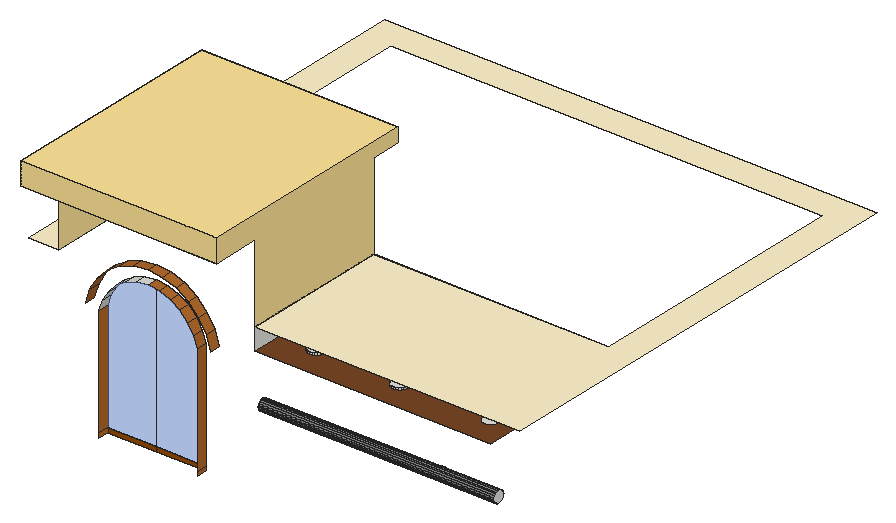
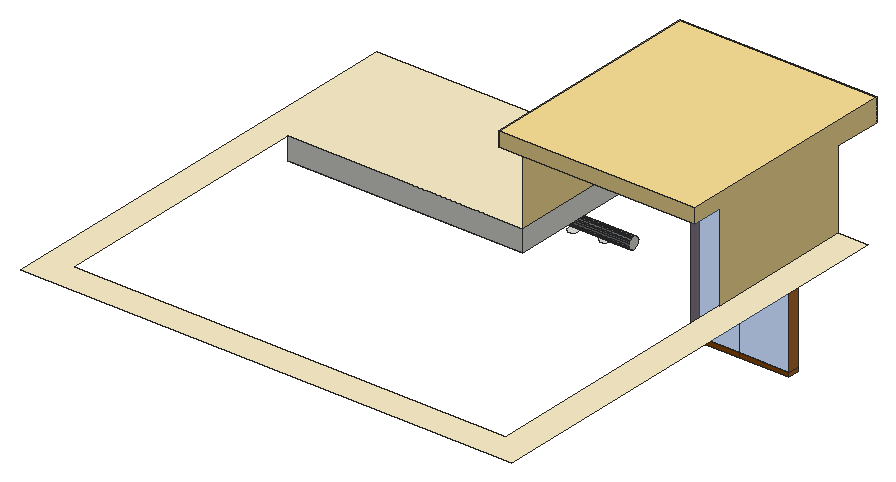
# SketchUp Ruby script. Lengths in inches.
U = 1.inch
M = Sketchup.active_model
def pt(a) = Geom::Point3d.new(a.map { |v| v * U })
def face(e, loops, mat)
  f = e.add_face(loops[0].map { |a| pt(a) })
  loops[1..].each { |l| e.add_face(l.map { |a| pt(a) }).erase! }
  f.material = f.back_material = mat if mat
  f
end
# faces: each face lists its corners as indices into pts; further lists are holes
def faces(e, pts, list, mat = nil) = list.each { |f| face(e, (f[0].is_a?(Array) ? f : [f]).map { |l| l.map { |i| pts[i] } }, mat) }
# xy, xz, yz: faces in a plane at the given z, y or x. An outline is a flat list of corners, or four numbers for a rectangle; further outlines are holes
def ring(l) = l.size == 4 ? [[l[0], l[1]], [l[2], l[1]], [l[2], l[3]], [l[0], l[3]]] : l.each_slice(2).to_a
def flat(e, list, mat, &to3) = list.each { |f| face(e, (f[0].is_a?(Array) ? f : [f]).map { |l| ring(l).map { |u, v| to3.(u, v) } }, mat) }
def xy(e, z, list, mat = nil) = flat(e, list, mat) { |x, y| [x, y, z] }
def xz(e, y, list, mat = nil) = flat(e, list, mat) { |x, z| [x, y, z] }
def yz(e, x, list, mat = nil) = flat(e, list, mat) { |y, z| [x, y, z] }
def lines(e, pts, list) = list.each { |a, b| e.add_line(pt(pts[a]), pt(pts[b])) }
# prism: a flat outline (further loops are holes) pulled along v
def prism(e, loops, v, mat = nil)
  f = face(e, loops, mat); d = Geom::Vector3d.new(v.map { |x| x * U })
  f.pushpull(f.normal.samedirection?(d) ? d.length : -d.length)
end
def box(e, o, s, mat = nil) = prism(e, [[o, [o[0] + s[0], o[1], o[2]], [o[0] + s[0], o[1] + s[1], o[2]], [o[0], o[1] + s[1], o[2]]]], [0, 0, s[2]], mat)
def at(x, y, z, deg = 0) = Geom::Transformation.translation(pt([x, y, z])) * Geom::Transformation.rotation(ORIGIN, Z_AXIS, deg.degrees)
def axes(o, x, y, z) = Geom::Transformation.new([*x, 0, *y, 0, *z, 0, *pt(o).to_a, 1])
def part(name) = M.definitions.add(name)
# library, detail: a bought-in or finely detailed component or shape, given as its bounding box
def library(name, o, s) = part(name).tap { |d| box(d.entities, o, s) }
def detail(e, o, s) = box(e.add_group.entities, o, s)
def put(e, d, t, mat = nil) = e.add_instance(d, t).tap { |i| i.material = mat if mat }
def group(e, t, mat = nil) = e.add_group.tap { |g| g.transformation = t; g.material = mat if mat }.entities
root = M.entities
M.materials.add("[Blacktop Old 01]").color = [132, 136, 139]
M.materials.add("[Color C07]").color = [153, 76, 0]
M.materials.add("[Color D01]").color = [255, 242, 204]
M.materials.add("[Color D02]").color = [255, 229, 153]
M.materials.add("[Translucent Glass Blue]").color = [100, 149, 237]
M.materials["[Translucent Glass Blue]"].alpha = 0.5
M.materials.add("[Wood Bamboo]").color = [177, 105, 43]
M.materials.add("[Wood Veneer 01]").color = [120, 70, 37]
xy(root,265.4375,[[117.93,77.67,118.3,77.72,118.65,77.86,118.94,78.09,119.17,78.39,119.32,78.73,119.36,79.11,119.32,79.48,119.17,79.83,118.94,80.12,118.65,80.35,118.3,80.5,117.93,80.54,117.56,80.5,117.21,80.35,116.91,80.12,116.68,79.83,116.54,79.48,116.49,79.11,116.54,78.73,116.68,78.39,116.91,78.09,117.21,77.86,117.56,77.72]])
xy(root,265.9375,[[129.74,77.67,130.11,77.72,130.46,77.86,130.76,78.09,130.98,78.39,131.13,78.73,131.18,79.11,131.13,79.48,130.98,79.83,130.76,80.12,130.46,80.35,130.11,80.5,129.74,80.54,129.37,80.5,129.02,80.35,128.72,80.12,128.49,79.83,128.35,79.48,128.3,79.11,128.35,78.73,128.49,78.39,128.72,78.09,129.02,77.86,129.37,77.72]])
xy(root,266.15,[[108.24,77.67,108.61,77.72,108.96,77.86,109.26,78.09,109.48,78.39,109.63,78.73,109.68,79.09,106.8,79.09,106.85,78.73,106.99,78.39,107.22,78.09,107.52,77.86,107.87,77.72],[106.8,79.09,109.68,79.09,109.68,79.11,109.63,79.48,109.48,79.83,109.26,80.12,108.96,80.35,108.61,80.5,108.24,80.54,107.87,80.5,107.52,80.35,107.22,80.12,106.99,79.83,106.85,79.48,106.8,79.11]])
xy(root,266.3125,[[141.86,77.67,142.24,77.72,142.58,77.86,142.88,78.09,143.11,78.39,143.25,78.73,143.3,79.11,143.25,79.48,143.11,79.83,142.88,80.12,142.58,80.35,142.24,80.5,141.86,80.54,141.49,80.5,141.15,80.35,140.85,80.12,140.62,79.83,140.48,79.48,140.43,79.11,140.48,78.73,140.62,78.39,140.85,78.09,141.15,77.86,141.49,77.72]])
xy(root,266.75,[[164.61,77.67,164.99,77.72,165.33,77.86,165.63,78.09,165.86,78.39,166,78.73,166.05,79.11,166,79.48,165.86,79.83,165.63,80.12,165.33,80.35,164.99,80.5,164.61,80.54,164.24,80.5,163.9,80.35,163.6,80.12,163.37,79.83,163.23,79.48,163.18,79.11,163.23,78.73,163.37,78.39,163.6,78.09,163.9,77.86,164.24,77.72]])
xy(root,267.84,[[153.24,77.67,153.61,77.72,153.96,77.86,154.26,78.09,154.48,78.39,154.63,78.73,154.68,79.11,154.63,79.48,154.6,79.54,151.88,79.54,151.85,79.48,151.8,79.11,151.85,78.73,151.99,78.39,152.22,78.09,152.52,77.86,152.87,77.72],[151.88,79.54,154.6,79.54,154.48,79.83,154.26,80.12,153.96,80.35,153.61,80.5,153.24,80.54,152.87,80.5,152.52,80.35,152.22,80.12,151.99,79.83]])
xy(root,283.17,[[165.02,81.32,164.35,81.41,163.73,81.66,163.2,82.07,162.8,82.6,162.54,83.22,162.45,83.88,162.54,84.55,162.8,85.16,163.2,85.69,163.73,86.1,164.35,86.36,165.02,86.44,165.68,86.36,166.3,86.1,166.83,85.69,167.24,85.16,167.49,84.55,167.58,83.88,167.49,83.22,167.24,82.6,166.83,82.07,166.3,81.66,165.68,81.41],[165.02,104.69,164.35,104.78,163.73,105.04,163.2,105.45,162.8,105.98,162.54,106.59,162.45,107.26,162.54,107.92,162.8,108.54,163.2,109.07,163.73,109.48,164.35,109.73,165.02,109.82,165.68,109.73,166.3,109.48,166.83,109.07,167.24,108.54,167.49,107.92,167.58,107.26,167.49,106.59,167.24,105.98,166.83,105.45,166.3,105.04,165.68,104.78]])
xy(root,283.17,[[[100.51,74.84,172.07,119.85],[165.02,104.69,165.68,104.78,166.3,105.04,166.83,105.45,167.24,105.98,167.49,106.59,167.58,107.26,167.49,107.92,167.24,108.54,166.83,109.07,166.3,109.48,165.68,109.73,165.02,109.82,164.35,109.73,163.73,109.48,163.2,109.07,162.8,108.54,162.54,107.92,162.45,107.26,162.54,106.59,162.8,105.98,163.2,105.45,163.73,105.04,164.35,104.78],[111.45,82.07,112.12,82.16,112.73,82.41,113.27,82.82,113.67,83.35,113.93,83.97,114.02,84.63,113.93,85.3,113.67,85.91,113.27,86.44,112.73,86.85,112.12,87.11,111.45,87.19,110.79,87.11,110.17,86.85,109.64,86.44,109.23,85.91,108.98,85.3,108.89,84.63,108.98,83.97,109.23,83.35,109.64,82.82,110.17,82.41,110.79,82.16],[111.45,104.69,112.12,104.78,112.73,105.04,113.27,105.45,113.67,105.98,113.93,106.59,114.02,107.26,113.93,107.92,113.67,108.54,113.27,109.07,112.73,109.48,112.12,109.73,111.45,109.82,110.79,109.73,110.17,109.48,109.64,109.07,109.23,108.54,108.98,107.92,108.89,107.26,108.98,106.59,109.23,105.98,109.64,105.45,110.17,105.04,110.79,104.78],[165.02,81.32,165.68,81.41,166.3,81.66,166.83,82.07,167.24,82.6,167.49,83.22,167.58,83.88,167.49,84.55,167.24,85.16,166.83,85.69,166.3,86.1,165.68,86.36,165.02,86.44,164.35,86.36,163.73,86.1,163.2,85.69,162.8,85.16,162.54,84.55,162.45,83.88,162.54,83.22,162.8,82.6,163.2,82.07,163.73,81.66,164.35,81.41],[137.45,81.32,138.12,81.41,138.73,81.66,139.27,82.07,139.67,82.6,139.93,83.22,140.02,83.88,139.93,84.55,139.67,85.16,139.27,85.69,138.73,86.1,138.12,86.36,137.45,86.44,136.79,86.36,136.17,86.1,135.64,85.69,135.23,85.16,134.98,84.55,134.89,83.88,134.98,83.22,135.23,82.6,135.64,82.07,136.17,81.66,136.79,81.41],[137.45,105.26,138.12,105.34,138.73,105.6,139.27,106.01,139.67,106.54,139.93,107.16,140.02,107.82,139.93,108.48,139.67,109.1,139.27,109.63,138.73,110.04,138.12,110.3,137.45,110.38,136.79,110.3,136.17,110.04,135.64,109.63,135.23,109.1,134.98,108.48,134.89,107.82,134.98,107.16,135.23,106.54,135.64,106.01,136.17,105.6,136.79,105.34]]],"[Wood Veneer 01]")
xy(root,283.61,[[137.45,81.32,136.79,81.41,136.17,81.66,135.64,82.07,135.23,82.6,134.98,83.22,134.89,83.88,134.98,84.55,135.23,85.16,135.64,85.69,136.17,86.1,136.79,86.36,137.45,86.44,138.12,86.36,138.73,86.1,139.27,85.69,139.67,85.16,139.93,84.55,140.02,83.88,139.93,83.22,139.67,82.6,139.27,82.07,138.73,81.66,138.12,81.41],[111.45,82.07,110.79,82.16,110.17,82.41,109.64,82.82,109.23,83.35,108.98,83.97,108.89,84.63,108.98,85.3,109.23,85.91,109.64,86.44,110.17,86.85,110.79,87.11,111.45,87.19,112.12,87.11,112.73,86.85,113.27,86.44,113.67,85.91,113.93,85.3,114.02,84.63,113.93,83.97,113.67,83.35,113.27,82.82,112.73,82.41,112.12,82.16],[111.45,104.69,110.79,104.78,110.17,105.04,109.64,105.45,109.23,105.98,108.98,106.59,108.89,107.26,108.98,107.92,109.23,108.54,109.64,109.07,110.17,109.48,110.79,109.73,111.45,109.82,112.12,109.73,112.73,109.48,113.27,109.07,113.67,108.54,113.93,107.92,114.02,107.26,113.93,106.59,113.67,105.98,113.27,105.45,112.73,105.04,112.12,104.78]])
xy(root,283.86,[[137.45,105.26,136.79,105.34,136.17,105.6,135.64,106.01,135.23,106.54,134.98,107.16,134.89,107.82,134.98,108.48,135.23,109.1,135.64,109.63,136.17,110.04,136.79,110.3,137.45,110.38,138.12,110.3,138.73,110.04,139.27,109.63,139.67,109.1,139.93,108.48,140.02,107.82,139.93,107.16,139.67,106.54,139.27,106.01,138.73,105.6,138.12,105.34]])
xy(root,289.8125,[[31.82,74.84,40.82,74.84,40.82,201.03,172.07,201.03,172.07,119.85,100.51,119.85,100.51,74.84,181.07,74.84,181.07,210.03,31.82,210.03]],"[Color D01]")
xy(root,313.4,[[40.82,60.4,100.51,74.84]])
xy(root,315.96,[[40.82,119.85,100.51,129.15]])
xy(root,320.375,[[40.82,60.4,100.51,129.15]],"[Color D02]")
xz(root,60.4,[[40.82,313.4,100.51,320.375]],"[Color D02]")
xz(root,74.84,[[55.76,245.31,70.65,246.56],[70.65,245.31,85.54,246.56]],"[Color C07]")
xz(root,74.84,[[55.76,246.56,70.65,246.56,70.65,292.04,67.19,291.64,63.91,290.47,60.98,288.58,58.5625,286.07,56.77,283.08,55.76,279.92],[70.65,246.56,85.54,246.56,85.54,279.92,84.53,283.08,82.74,286.07,80.32,288.58,77.39,290.47,74.11,291.64,70.65,292.04]],"[Translucent Glass Blue]")
xz(root,119.85,[[100.51,283.17,172.07,289.8125]])
xz(root,129.15,[[40.82,315.96,100.51,320.375]],"[Color D02]")
yz(root,40.82,[[74.84,289.8125,119.85,289.8125,119.85,315.96,129.15,315.96,129.15,320.375,60.4,320.375,60.4,313.4,74.84,313.4]],"[Color D02]")
yz(root,55.76,[[71.71,245.31,74.84,246.56],[71.71,246.56,74.84,279.92]],"[Wood Bamboo]")
yz(root,85.54,[[71.71,245.31,74.84,246.56],[71.71,246.56,74.84,279.92]],"[Wood Bamboo]")
yz(root,100.51,[[77.85,265.64,77.4,265.7,76.98,265.87,76.62,266.15,76.34,266.51,76.16,266.93,76.1,267.39,76.16,267.84,76.34,268.26,76.62,268.625,76.98,268.9,77.4,269.08,77.85,269.14,78.31,269.08,78.73,268.9,79.09,268.625,79.37,268.26,79.54,267.84,79.6,267.39,79.54,266.93,79.37,266.51,79.09,266.15,78.73,265.87,78.31,265.7],[74.84,283.17,119.85,289.8125]])
yz(root,100.51,[[74.84,289.8125,119.85,289.8125,119.85,315.96,129.15,315.96,129.15,320.375,60.4,320.375,60.4,313.4,74.84,313.4]],"[Color D02]")
yz(root,172.14,[[77.85,265.64,78.31,265.7,78.73,265.87,79.09,266.15,79.37,266.51,79.54,266.93,79.6,267.39,79.54,267.84,79.37,268.26,79.09,268.625,78.73,268.9,78.31,269.08,77.85,269.14,77.4,269.08,76.98,268.9,76.62,268.625,76.34,268.26,76.16,267.84,76.1,267.39,76.16,266.93,76.34,266.51,76.62,266.15,76.98,265.87,77.4,265.7]])
p = [[100.51,77.4,265.7],[100.51,77.85,265.64],[172.14,77.85,265.64],[172.14,77.4,265.7],[100.51,78.31,265.7],[172.14,78.31,265.7],
  [100.51,76.98,265.87],[172.14,76.98,265.87],[100.51,78.73,265.87],[172.14,78.73,265.87],[100.51,76.62,266.15],[172.14,76.62,266.15],
  [100.51,79.09,266.15],[106.8,79.09,266.15],[109.68,79.09,266.15],[172.14,79.09,266.15],[100.51,76.34,266.51],[172.14,76.34,266.51],
  [100.51,79.37,266.51],[172.14,79.37,266.51],[100.51,76.16,266.93],[172.14,76.16,266.93],[100.51,79.54,266.93],[172.14,79.54,266.93],
  [100.51,76.1,267.39],[172.14,76.1,267.39],[100.51,79.6,267.39],[172.14,79.6,267.39],[100.51,76.16,267.84],[172.14,76.16,267.84],
  [100.51,79.54,267.84],[151.88,79.54,267.84],[154.6,79.54,267.84],[172.14,79.54,267.84],[100.51,76.34,268.26],[172.14,76.34,268.26],
  [100.51,79.37,268.26],[172.14,79.37,268.26],[100.51,76.62,268.625],[172.14,76.62,268.625],[100.51,79.09,268.625],[172.14,79.09,268.625],
  [100.51,76.98,268.9],[172.14,76.98,268.9],[100.51,78.73,268.9],[172.14,78.73,268.9],[100.51,77.4,269.08],[172.14,77.4,269.08],
  [100.51,78.31,269.08],[172.14,78.31,269.08],[100.51,77.85,269.14],[172.14,77.85,269.14],[55.76,74.84,279.92],[56.77,74.84,283.08],
  [56.77,71.71,283.08],[55.76,71.71,279.92],[84.53,74.84,283.08],[85.54,74.84,279.92],[85.54,71.71,279.92],[84.53,71.71,283.08],
  [53,74.84,284.79],[51.65,74.84,280.57],[51.65,71.71,280.57],[53,71.71,284.79],[89.65,74.84,280.57],[88.3,74.84,284.79],
  [88.3,71.71,284.79],[89.65,71.71,280.57],[58.5625,74.84,286.07],[58.5625,71.71,286.07],[82.74,74.84,286.07],[82.74,71.71,286.07],
  [137.45,81.32,283.17],[136.79,81.41,283.17],[136.79,81.41,283.61],[137.45,81.32,283.61],[138.12,81.41,283.17],[138.12,81.41,283.61],
  [136.17,81.66,283.17],[136.17,81.66,283.61],[138.73,81.66,283.17],[138.73,81.66,283.61],[135.64,82.07,283.17],[135.64,82.07,283.61],
  [139.27,82.07,283.17],[139.27,82.07,283.61],[111.45,82.07,283.17],[110.79,82.16,283.17],[110.79,82.16,283.61],[111.45,82.07,283.61],
  [112.12,82.16,283.17],[112.12,82.16,283.61],[135.23,82.6,283.17],[135.23,82.6,283.61],[139.67,82.6,283.17],[139.67,82.6,283.61],
  [110.17,82.41,283.17],[110.17,82.41,283.61],[112.73,82.41,283.17],[112.73,82.41,283.61],[109.64,82.82,283.17],[109.64,82.82,283.61],
  [113.27,82.82,283.17],[113.27,82.82,283.61],[134.98,83.22,283.17],[134.98,83.22,283.61],[139.93,83.22,283.17],[139.93,83.22,283.61],
  [109.23,83.35,283.17],[109.23,83.35,283.61],[113.67,83.35,283.17],[113.67,83.35,283.61],[134.89,83.88,283.17],[134.89,83.88,283.61],
  [140.02,83.88,283.17],[140.02,83.88,283.61],[108.98,83.97,283.17],[108.98,83.97,283.61],[113.93,83.97,283.17],[113.93,83.97,283.61],
  [134.98,84.55,283.17],[134.98,84.55,283.61],[139.93,84.55,283.17],[139.93,84.55,283.61],[108.89,84.63,283.17],[108.89,84.63,283.61],
  [114.02,84.63,283.17],[114.02,84.63,283.61],[135.23,85.16,283.17],[135.23,85.16,283.61],[139.67,85.16,283.17],[139.67,85.16,283.61],
  [108.98,85.3,283.17],[108.98,85.3,283.61],[113.93,85.3,283.17],[113.93,85.3,283.61],[135.64,85.69,283.17],[135.64,85.69,283.61],
  [139.27,85.69,283.17],[139.27,85.69,283.61],[109.23,85.91,283.17],[109.23,85.91,283.61],[113.67,85.91,283.17],[113.67,85.91,283.61],
  [136.17,86.1,283.17],[136.17,86.1,283.61],[138.73,86.1,283.17],[138.73,86.1,283.61],[109.64,86.44,283.17],[109.64,86.44,283.61],
  [113.27,86.44,283.17],[113.27,86.44,283.61],[136.79,86.36,283.17],[136.79,86.36,283.61],[138.12,86.36,283.17],[138.12,86.36,283.61],
  [110.17,86.85,283.17],[110.17,86.85,283.61],[112.73,86.85,283.17],[112.73,86.85,283.61],[137.45,86.44,283.17],[137.45,86.44,283.61],
  [110.79,87.11,283.17],[110.79,87.11,283.61],[112.12,87.11,283.17],[112.12,87.11,283.61],[111.45,87.19,283.17],[111.45,87.19,283.61],
  [111.45,104.69,283.17],[110.79,104.78,283.17],[110.79,104.78,283.61],[111.45,104.69,283.61],[112.12,104.78,283.17],[112.12,104.78,283.61],
  [110.17,105.04,283.17],[110.17,105.04,283.61],[112.73,105.04,283.17],[112.73,105.04,283.61],[109.64,105.45,283.17],[109.64,105.45,283.61],
  [113.27,105.45,283.17],[113.27,105.45,283.61],[136.79,105.34,283.17],[136.17,105.6,283.17],[136.17,105.6,283.86],[136.79,105.34,283.86],
  [137.45,105.26,283.17],[137.45,105.26,283.86],[138.12,105.34,283.17],[138.12,105.34,283.86],[138.73,105.6,283.17],[138.73,105.6,283.86],
  [109.23,105.98,283.17],[109.23,105.98,283.61],[113.67,105.98,283.17],[113.67,105.98,283.61],[135.64,106.01,283.17],[135.64,106.01,283.86],
  [139.27,106.01,283.17],[139.27,106.01,283.86],[108.98,106.59,283.17],[108.98,106.59,283.61],[113.93,106.59,283.17],[113.93,106.59,283.61],
  [135.23,106.54,283.17],[135.23,106.54,283.86],[139.67,106.54,283.17],[139.67,106.54,283.86],[134.98,107.16,283.17],[134.98,107.16,283.86],
  [139.93,107.16,283.17],[139.93,107.16,283.86],[108.89,107.26,283.17],[108.89,107.26,283.61],[114.02,107.26,283.17],[114.02,107.26,283.61],
  [134.89,107.82,283.17],[134.89,107.82,283.86],[140.02,107.82,283.17],[140.02,107.82,283.86],[108.98,107.92,283.17],[108.98,107.92,283.61],
  [113.93,107.92,283.17],[113.93,107.92,283.61],[134.98,108.48,283.17],[134.98,108.48,283.86],[139.93,108.48,283.17],[139.93,108.48,283.86],
  [109.23,108.54,283.17],[109.23,108.54,283.61],[113.67,108.54,283.17],[113.67,108.54,283.61],[109.64,109.07,283.17],[109.64,109.07,283.61],
  [113.27,109.07,283.17],[113.27,109.07,283.61],[135.23,109.1,283.17],[135.23,109.1,283.86],[139.67,109.1,283.17],[139.67,109.1,283.86],
  [110.17,109.48,283.17],[110.17,109.48,283.61],[112.73,109.48,283.17],[112.73,109.48,283.61],[135.64,109.63,283.17],[135.64,109.63,283.86],
  [139.27,109.63,283.17],[139.27,109.63,283.86],[110.79,109.73,283.17],[110.79,109.73,283.61],[112.12,109.73,283.17],[112.12,109.73,283.61],
  [136.17,110.04,283.17],[136.17,110.04,283.86],[138.73,110.04,283.17],[138.73,110.04,283.86],[111.45,109.82,283.17],[111.45,109.82,283.61],
  [136.79,110.3,283.17],[136.79,110.3,283.86],[138.12,110.3,283.17],[138.12,110.3,283.86],[137.45,110.38,283.17],[137.45,110.38,283.86],
  [55.28,74.84,288.59],[55.28,71.71,288.59],[86.03,74.84,288.59],[86.03,71.71,288.59],[60.98,74.84,288.58],[60.98,71.71,288.58],
  [80.32,74.84,288.58],[80.32,71.71,288.58],[58.35,74.84,291.78],[58.35,71.71,291.78],[63.91,74.84,290.47],[63.91,71.71,290.47],
  [77.39,74.84,290.47],[77.39,71.71,290.47],[82.95,74.84,291.78],[82.95,71.71,291.78],[67.19,74.84,291.64],[67.19,71.71,291.64],
  [74.11,74.84,291.64],[74.11,71.71,291.64],[70.65,74.84,292.04],[70.65,71.71,292.04],[62.08,74.84,294.18],[62.08,71.71,294.18],
  [79.23,74.84,294.18],[79.23,71.71,294.18],[66.25,74.84,295.68],[66.25,71.71,295.68],[75.05,74.84,295.68],[75.05,71.71,295.68],
  [70.65,74.84,296.18],[70.65,71.71,296.18]]
faces(root,p,[[0,1,2,3],[1,4,5,2],[6,0,3,7],[4,8,9,5],[10,6,7,11],[8,12,13,14,15,9],[16,10,11,17],[12,18,19,15,14,13],
  [20,16,17,21],[18,22,23,19],[24,20,21,25],[22,26,27,23],[28,24,25,29],[26,30,31,32,33,27],[34,28,29,35],[30,36,37,33,32,31],
  [38,34,35,39],[36,40,41,37],[42,38,39,43],[40,44,45,41],[46,42,43,47],[44,48,49,45],[50,46,47,51],[48,50,51,49]],"[Blacktop Old 01]")
faces(root,p,[[52,53,54,55],[53,68,69,54],[72,73,74,75],[76,72,75,77],[73,78,79,74],[80,76,77,81],[78,82,83,79],[84,80,81,85],
  [86,87,88,89],[90,86,89,91],[82,92,93,83],[94,84,85,95],[87,96,97,88],[98,90,91,99],[96,100,101,97],[102,98,99,103],
  [92,104,105,93],[106,94,95,107],[100,108,109,101],[110,102,103,111],[104,112,113,105],[114,106,107,115],[108,116,117,109],[118,110,111,119],
  [112,120,121,113],[122,114,115,123],[116,124,125,117],[126,118,119,127],[120,128,129,121],[130,122,123,131],[124,132,133,125],[134,126,127,135],
  [128,136,137,129],[138,130,131,139],[132,140,141,133],[142,134,135,143],[136,144,145,137],[146,138,139,147],[140,148,149,141],[150,142,143,151],
  [144,152,153,145],[154,146,147,155],[148,156,157,149],[158,150,151,159],[152,160,161,153],[160,154,155,161],[156,162,163,157],[164,158,159,165],
  [162,166,167,163],[166,164,165,167],[168,169,170,171],[172,168,171,173],[169,174,175,170],[176,172,173,177],[174,178,179,175],[180,176,177,181],
  [182,183,184,185],[186,182,185,187],[188,186,187,189],[190,188,189,191],[178,192,193,179],[194,180,181,195],[183,196,197,184],[198,190,191,199],
  [192,200,201,193],[202,194,195,203],[196,204,205,197],[206,198,199,207],[204,208,209,205],[210,206,207,211],[200,212,213,201],[214,202,203,215],
  [208,216,217,209],[218,210,211,219],[212,220,221,213],[222,214,215,223],[216,224,225,217],[226,218,219,227],[220,228,229,221],[230,222,223,231],
  [228,232,233,229],[234,230,231,235],[224,236,237,225],[238,226,227,239],[232,240,241,233],[242,234,235,243],[236,244,245,237],[246,238,239,247],
  [240,248,249,241],[250,242,243,251],[244,252,253,245],[254,246,247,255],[248,256,257,249],[256,250,251,257],[252,258,259,253],[260,254,255,261],
  [258,262,263,259],[262,260,261,263],[68,268,269,69],[268,274,275,269],[274,280,281,275],[280,284,285,281]])
faces(root,p,[[56,57,58,59],[60,61,62,63],[64,65,66,67],[70,56,59,71],[264,60,63,265],[65,266,267,66],[270,70,71,271],[272,264,265,273],
  [276,270,271,277],[266,278,279,267],[282,276,277,283],[284,282,283,285],[286,272,273,287],[278,288,289,279],[290,286,287,291],[288,292,293,289],
  [294,290,291,295],[292,294,295,293]],"[Wood Bamboo]")
